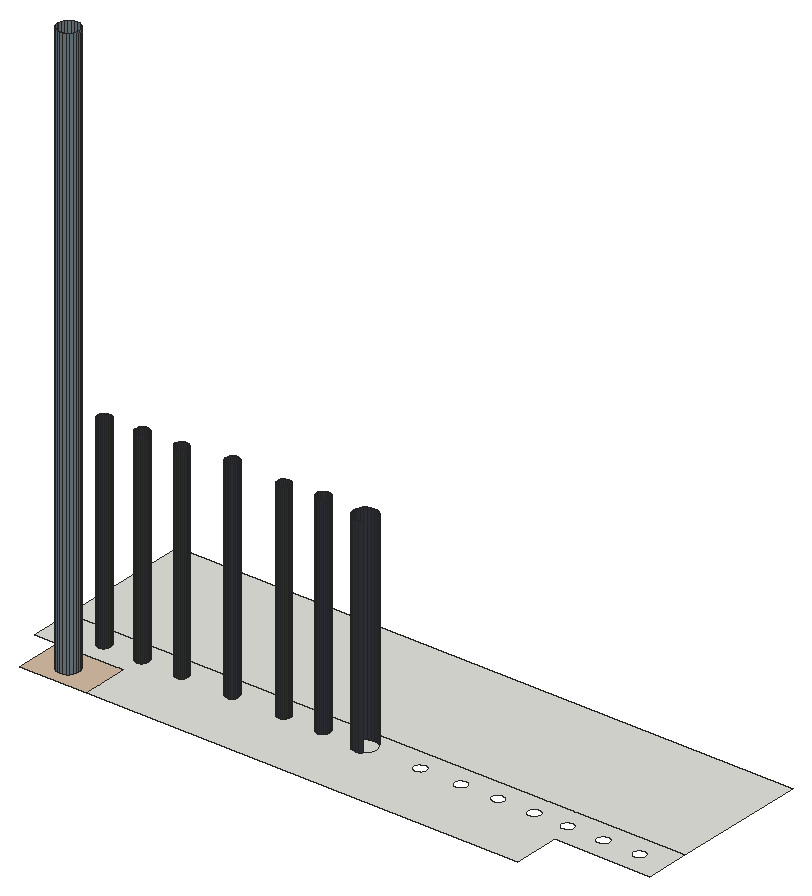
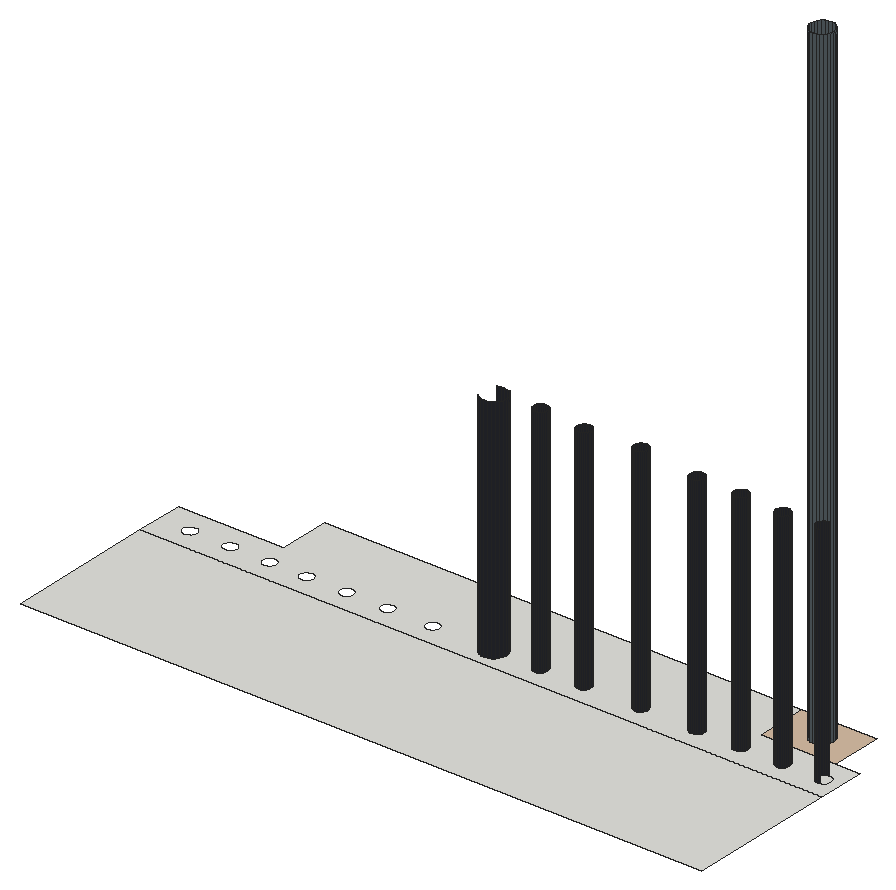
# SketchUp Ruby script. Lengths in inches.
U = 1.inch
M = Sketchup.active_model
def pt(a) = Geom::Point3d.new(a.map { |v| v * U })
def face(e, loops, mat)
  f = e.add_face(loops[0].map { |a| pt(a) })
  loops[1..].each { |l| e.add_face(l.map { |a| pt(a) }).erase! }
  f.material = f.back_material = mat if mat
  f
end
# faces: each face lists its corners as indices into pts; further lists are holes
def faces(e, pts, list, mat = nil) = list.each { |f| face(e, (f[0].is_a?(Array) ? f : [f]).map { |l| l.map { |i| pts[i] } }, mat) }
# xy, xz, yz: faces in a plane at the given z, y or x. An outline is a flat list of corners, or four numbers for a rectangle; further outlines are holes
def ring(l) = l.size == 4 ? [[l[0], l[1]], [l[2], l[1]], [l[2], l[3]], [l[0], l[3]]] : l.each_slice(2).to_a
def flat(e, list, mat, &to3) = list.each { |f| face(e, (f[0].is_a?(Array) ? f : [f]).map { |l| ring(l).map { |u, v| to3.(u, v) } }, mat) }
def xy(e, z, list, mat = nil) = flat(e, list, mat) { |x, y| [x, y, z] }
def xz(e, y, list, mat = nil) = flat(e, list, mat) { |x, z| [x, y, z] }
def yz(e, x, list, mat = nil) = flat(e, list, mat) { |y, z| [x, y, z] }
def lines(e, pts, list) = list.each { |a, b| e.add_line(pt(pts[a]), pt(pts[b])) }
# prism: a flat outline (further loops are holes) pulled along v
def prism(e, loops, v, mat = nil)
  f = face(e, loops, mat); d = Geom::Vector3d.new(v.map { |x| x * U })
  f.pushpull(f.normal.samedirection?(d) ? d.length : -d.length)
end
def box(e, o, s, mat = nil) = prism(e, [[o, [o[0] + s[0], o[1], o[2]], [o[0] + s[0], o[1] + s[1], o[2]], [o[0], o[1] + s[1], o[2]]]], [0, 0, s[2]], mat)
def at(x, y, z, deg = 0) = Geom::Transformation.translation(pt([x, y, z])) * Geom::Transformation.rotation(ORIGIN, Z_AXIS, deg.degrees)
def axes(o, x, y, z) = Geom::Transformation.new([*x, 0, *y, 0, *z, 0, *pt(o).to_a, 1])
def part(name) = M.definitions.add(name)
# library, detail: a bought-in or finely detailed component or shape, given as its bounding box
def library(name, o, s) = part(name).tap { |d| box(d.entities, o, s) }
def detail(e, o, s) = box(e.add_group.entities, o, s)
def put(e, d, t, mat = nil) = e.add_instance(d, t).tap { |i| i.material = mat if mat }
def group(e, t, mat = nil) = e.add_group.tap { |g| g.transformation = t; g.material = mat if mat }.entities
root = M.entities
M.materials.add("[Formica Laminate Dark]").color = [50, 53, 60]
M.materials.add("[Formica Laminate Light]").color = [213, 189, 164]
M.materials.add("[Formica Speckled Grey]").color = [112, 125, 132]
xy(root,479.47,[[[305.49,83.42,364.3,83.42,364.3,89.73,377.32,89.73,377.32,95.64,293.32,95.64,293.32,89.73,305.49,89.73],[335.9,91.32,335.49,91.37,335.11,91.53,334.79,91.78,334.54,92.1,334.39,92.48,334.33,92.88,334.39,93.28,334.54,93.66,334.79,93.99,335.11,94.23,335.49,94.39,335.9,94.44,336.3,94.39,336.68,94.23,337,93.99,337.25,93.66,337.41,93.28,337.46,92.88,337.41,92.48,337.25,92.1,337,91.78,336.68,91.53,336.3,91.37],[317.9,91.9,317.68,91.93,317.47,92.02,317.28,92.16,317.15,92.34,317.06,92.55,317.03,92.78,317.06,93.01,317.15,93.22,317.28,93.4,317.47,93.54,317.68,93.625,317.9,93.65,318.13,93.625,318.34,93.54,318.52,93.4,318.66,93.22,318.75,93.01,318.78,92.78,318.75,92.55,318.66,92.34,318.52,92.16,318.34,92.02,318.13,91.93],[343.53,91.9,343.3,91.93,343.09,92.02,342.91,92.16,342.77,92.34,342.68,92.55,342.65,92.78,342.68,93.01,342.77,93.22,342.91,93.4,343.09,93.54,343.3,93.625,343.53,93.65,343.75,93.625,343.97,93.54,344.15,93.4,344.29,93.22,344.375,93.01,344.4,92.78,344.375,92.55,344.29,92.34,344.15,92.16,343.97,92.02,343.75,91.93],[373.47,91.9,373.24,91.93,373.03,92.02,372.85,92.16,372.71,92.34,372.62,92.55,372.59,92.78,372.62,93.01,372.71,93.22,372.85,93.4,373.03,93.54,373.24,93.625,373.47,93.65,373.69,93.625,373.9,93.54,374.08,93.4,374.22,93.22,374.3125,93.01,374.34,92.78,374.3125,92.55,374.22,92.34,374.08,92.16,373.9,92.02,373.69,91.93],[349.09,91.9,348.86,91.93,348.65,92.02,348.47,92.16,348.33,92.34,348.25,92.55,348.22,92.78,348.25,93.01,348.33,93.22,348.47,93.4,348.65,93.54,348.86,93.625,349.09,93.65,349.32,93.625,349.53,93.54,349.71,93.4,349.85,93.22,349.9375,93.01,349.97,92.78,349.9375,92.55,349.85,92.34,349.71,92.16,349.53,92.02,349.32,91.93],[368.53,91.9,368.3,91.93,368.09,92.02,367.91,92.16,367.77,92.34,367.68,92.55,367.65,92.78,367.68,93.01,367.77,93.22,367.91,93.4,368.09,93.54,368.3,93.625,368.53,93.65,368.75,93.625,368.97,93.54,369.15,93.4,369.29,93.22,369.375,93.01,369.4,92.78,369.375,92.55,369.29,92.34,369.15,92.16,368.97,92.02,368.75,91.93],[354.15,91.9,353.93,91.93,353.72,92.02,353.53,92.16,353.4,92.34,353.31,92.55,353.28,92.78,353.31,93.01,353.4,93.22,353.53,93.4,353.72,93.54,353.93,93.625,354.15,93.65,354.38,93.625,354.59,93.54,354.77,93.4,354.91,93.22,355,93.01,355.03,92.78,355,92.55,354.91,92.34,354.77,92.16,354.59,92.02,354.38,91.93],[363.65,91.9,363.43,91.93,363.22,92.02,363.03,92.16,362.9,92.34,362.81,92.55,362.78,92.78,362.81,93.01,362.9,93.22,363.03,93.4,363.22,93.54,363.43,93.625,363.65,93.65,363.88,93.625,364.09,93.54,364.27,93.4,364.41,93.22,364.5,93.01,364.53,92.78,364.5,92.55,364.41,92.34,364.27,92.16,364.09,92.02,363.88,91.93],[359.09,91.9,358.86,91.93,358.65,92.02,358.47,92.16,358.33,92.34,358.25,92.55,358.22,92.78,358.25,93.01,358.33,93.22,358.47,93.4,358.65,93.54,358.86,93.625,359.09,93.65,359.32,93.625,359.53,93.54,359.71,93.4,359.85,93.22,359.9375,93.01,359.97,92.78,359.9375,92.55,359.85,92.34,359.71,92.16,359.53,92.02,359.32,91.93],[295.4,91.9,295.18,91.93,294.97,92.02,294.78,92.16,294.65,92.34,294.56,92.55,294.53,92.78,294.56,93.01,294.65,93.22,294.78,93.4,294.97,93.54,295.18,93.625,295.4,93.65,295.63,93.625,295.84,93.54,296.02,93.4,296.16,93.22,296.25,93.01,296.28,92.78,296.25,92.55,296.16,92.34,296.02,92.16,295.84,92.02,295.63,91.93],[330.28,91.9,330.05,91.93,329.84,92.02,329.66,92.16,329.52,92.34,329.43,92.55,329.4,92.78,329.43,93.01,329.52,93.22,329.66,93.4,329.84,93.54,330.05,93.625,330.28,93.65,330.5,93.625,330.72,93.54,330.9,93.4,331.04,93.22,331.125,93.01,331.15,92.78,331.125,92.55,331.04,92.34,330.9,92.16,330.72,92.02,330.5,91.93],[300.4,91.9,300.18,91.93,299.97,92.02,299.78,92.16,299.65,92.34,299.56,92.55,299.53,92.78,299.56,93.01,299.65,93.22,299.78,93.4,299.97,93.54,300.18,93.625,300.4,93.65,300.63,93.625,300.84,93.54,301.02,93.4,301.16,93.22,301.25,93.01,301.28,92.78,301.25,92.55,301.16,92.34,301.02,92.16,300.84,92.02,300.63,91.93],[324.9,91.9,324.68,91.93,324.47,92.02,324.28,92.16,324.15,92.34,324.06,92.55,324.03,92.78,324.06,93.01,324.15,93.22,324.28,93.4,324.47,93.54,324.68,93.625,324.9,93.65,325.13,93.625,325.34,93.54,325.52,93.4,325.66,93.22,325.75,93.01,325.78,92.78,325.75,92.55,325.66,92.34,325.52,92.16,325.34,92.02,325.13,91.93],[305.59,91.9,305.36,91.93,305.15,92.02,304.97,92.16,304.83,92.34,304.75,92.55,304.72,92.78,304.75,93.01,304.83,93.22,304.97,93.4,305.15,93.54,305.36,93.625,305.59,93.65,305.82,93.625,306.03,93.54,306.21,93.4,306.35,93.22,306.4375,93.01,306.47,92.78,306.4375,92.55,306.35,92.34,306.21,92.16,306.03,92.02,305.82,91.93],[310.97,91.9,310.74,91.93,310.53,92.02,310.35,92.16,310.21,92.34,310.12,92.55,310.09,92.78,310.12,93.01,310.21,93.22,310.35,93.4,310.53,93.54,310.74,93.625,310.97,93.65,311.19,93.625,311.4,93.54,311.58,93.4,311.72,93.22,311.8125,93.01,311.84,92.78,311.8125,92.55,311.72,92.34,311.58,92.16,311.4,92.02,311.19,91.93]],[300.64,84.97,300.26,85.02,299.92,85.17,299.62,85.4,299.39,85.69,299.25,86.04,299.2,86.41,299.25,86.78,299.39,87.13,299.62,87.43,299.92,87.66,300.26,87.8,300.64,87.85,301.01,87.8,301.36,87.66,301.65,87.43,301.88,87.13,302.03,86.78,302.07,86.41,302.03,86.04,301.88,85.69,301.65,85.4,301.36,85.17,301.01,85.02],[335.9,91.32,335.49,91.37,335.11,91.53,334.79,91.78,334.54,92.1,334.39,92.48,334.33,92.88,334.39,93.28,334.54,93.66,334.79,93.99,335.11,94.23,335.49,94.39,335.9,94.44,336.3,94.39,336.68,94.23,337,93.99,337.25,93.66,337.41,93.28,337.46,92.88,337.41,92.48,337.25,92.1,337,91.78,336.68,91.53,336.3,91.37],[295.4,91.9,295.18,91.93,294.97,92.02,294.78,92.16,294.65,92.34,294.56,92.55,294.53,92.78,294.56,93.01,294.65,93.22,294.78,93.4,294.97,93.54,295.18,93.625,295.4,93.65,295.63,93.625,295.84,93.54,296.02,93.4,296.16,93.22,296.25,93.01,296.28,92.78,296.25,92.55,296.16,92.34,296.02,92.16,295.84,92.02,295.63,91.93],[300.4,91.9,300.18,91.93,299.97,92.02,299.78,92.16,299.65,92.34,299.56,92.55,299.53,92.78,299.56,93.01,299.65,93.22,299.78,93.4,299.97,93.54,300.18,93.625,300.4,93.65,300.63,93.625,300.84,93.54,301.02,93.4,301.16,93.22,301.25,93.01,301.28,92.78,301.25,92.55,301.16,92.34,301.02,92.16,300.84,92.02,300.63,91.93],
  [305.59,91.9,305.36,91.93,305.15,92.02,304.97,92.16,304.83,92.34,304.75,92.55,304.72,92.78,304.75,93.01,304.83,93.22,304.97,93.4,305.15,93.54,305.36,93.625,305.59,93.65,305.82,93.625,306.03,93.54,306.21,93.4,306.35,93.22,306.4375,93.01,306.47,92.78,306.4375,92.55,306.35,92.34,306.21,92.16,306.03,92.02,305.82,91.93],[310.97,91.9,310.74,91.93,310.53,92.02,310.35,92.16,310.21,92.34,310.12,92.55,310.09,92.78,310.12,93.01,310.21,93.22,310.35,93.4,310.53,93.54,310.74,93.625,310.97,93.65,311.19,93.625,311.4,93.54,311.58,93.4,311.72,93.22,311.8125,93.01,311.84,92.78,311.8125,92.55,311.72,92.34,311.58,92.16,311.4,92.02,311.19,91.93],[317.9,91.9,317.68,91.93,317.47,92.02,317.28,92.16,317.15,92.34,317.06,92.55,317.03,92.78,317.06,93.01,317.15,93.22,317.28,93.4,317.47,93.54,317.68,93.625,317.9,93.65,318.13,93.625,318.34,93.54,318.52,93.4,318.66,93.22,318.75,93.01,318.78,92.78,318.75,92.55,318.66,92.34,318.52,92.16,318.34,92.02,318.13,91.93],[324.9,91.9,324.68,91.93,324.47,92.02,324.28,92.16,324.15,92.34,324.06,92.55,324.03,92.78,324.06,93.01,324.15,93.22,324.28,93.4,324.47,93.54,324.68,93.625,324.9,93.65,325.13,93.625,325.34,93.54,325.52,93.4,325.66,93.22,325.75,93.01,325.78,92.78,325.75,92.55,325.66,92.34,325.52,92.16,325.34,92.02,325.13,91.93],[330.28,91.9,330.05,91.93,329.84,92.02,329.66,92.16,329.52,92.34,329.43,92.55,329.4,92.78,329.43,93.01,329.52,93.22,329.66,93.4,329.84,93.54,330.05,93.625,330.28,93.65,330.5,93.625,330.72,93.54,330.9,93.4,331.04,93.22,331.125,93.01,331.15,92.78,331.125,92.55,331.04,92.34,330.9,92.16,330.72,92.02,330.5,91.93],
  [293.32,95.64,377.32,114.1]])
xy(root,479.47,[[[296.37,83.42,305.49,89.73],[300.64,84.97,300.26,85.02,299.92,85.17,299.62,85.4,299.39,85.69,299.25,86.04,299.2,86.41,299.25,86.78,299.39,87.13,299.62,87.43,299.92,87.66,300.26,87.8,300.64,87.85,301.01,87.8,301.36,87.66,301.65,87.43,301.88,87.13,302.03,86.78,302.07,86.41,302.03,86.04,301.88,85.69,301.65,85.4,301.36,85.17,301.01,85.02]]],"[Formica Laminate Light]")
p = [[299.92,85.17,479.47],[300.26,85.02,479.47],[300.26,85.02,557.86],[299.92,85.17,557.86],[300.64,84.97,479.47],[300.64,84.97,557.86],
  [301.01,85.02,479.47],[301.01,85.02,557.86],[301.36,85.17,479.47],[301.36,85.17,557.86],[299.62,85.4,479.47],[299.62,85.4,557.86],
  [301.65,85.4,479.47],[301.65,85.4,557.86],[299.39,85.69,479.47],[299.39,85.69,557.86],[301.88,85.69,479.47],[301.88,85.69,557.86],
  [299.25,86.04,479.47],[299.25,86.04,557.86],[302.03,86.04,479.47],[302.03,86.04,557.86],[299.2,86.41,479.47],[299.2,86.41,557.86],
  [302.07,86.41,479.47],[302.07,86.41,557.86],[299.25,86.78,479.47],[299.25,86.78,557.86],[302.03,86.78,479.47],[302.03,86.78,557.86],
  [299.39,87.13,479.47],[299.39,87.13,557.86],[301.88,87.13,479.47],[301.88,87.13,557.86],[299.62,87.43,479.47],[299.62,87.43,557.86],
  [301.65,87.43,479.47],[301.65,87.43,557.86],[299.92,87.66,479.47],[299.92,87.66,557.86],[301.36,87.66,479.47],[301.36,87.66,557.86],
  [300.26,87.8,479.47],[300.26,87.8,557.86],[301.01,87.8,479.47],[301.01,87.8,557.86],[300.64,87.85,479.47],[300.64,87.85,557.86],
  [335.49,91.37,479.47],[335.9,91.32,479.47],[335.9,91.32,507.81],[335.49,91.37,507.81],[336.3,91.37,479.47],[336.3,91.37,507.81],
  [335.11,91.53,479.47],[335.11,91.53,507.81],[336.68,91.53,479.47],[336.68,91.53,507.81],[334.79,91.78,479.47],[334.79,91.78,507.81],
  [334.54,92.1,479.47],[334.54,92.1,507.81],[295.4,91.9,479.47],[295.63,91.93,479.47],[295.63,91.93,507.47],[295.4,91.9,507.47],
  [295.84,92.02,479.47],[295.84,92.02,507.47],[299.97,92.02,479.47],[300.18,91.93,479.47],[300.18,91.93,507.22],[299.97,92.02,507.22],
  [300.4,91.9,479.47],[300.4,91.9,507.22],[300.63,91.93,479.47],[300.63,91.93,507.22],[300.84,92.02,479.47],[300.84,92.02,507.22],
  [305.15,92.02,479.47],[305.36,91.93,479.47],[305.36,91.93,507.41],[305.15,92.02,507.41],[305.59,91.9,479.47],[305.59,91.9,507.41],
  [305.82,91.93,479.47],[305.82,91.93,507.41],[306.03,92.02,479.47],[306.03,92.02,507.41],[310.53,92.02,479.47],[310.74,91.93,479.47],
  [310.74,91.93,507.47],[310.53,92.02,507.47],[310.97,91.9,479.47],[310.97,91.9,507.47],[311.19,91.93,479.47],[311.19,91.93,507.47],
  [311.4,92.02,479.47],[311.4,92.02,507.47],[317.47,92.02,479.47],[317.68,91.93,479.47],[317.68,91.93,508.19],[317.47,92.02,508.19],
  [317.9,91.9,479.47],[317.9,91.9,508.19],[318.13,91.93,479.47],[318.13,91.93,508.19],[318.34,92.02,479.47],[318.34,92.02,508.19],
  [324.47,92.02,479.47],[324.68,91.93,479.47],[324.68,91.93,507.81],[324.47,92.02,507.81],[324.9,91.9,479.47],[324.9,91.9,507.81],
  [325.13,91.93,479.47],[325.13,91.93,507.81],[325.34,92.02,479.47],[325.34,92.02,507.81],[329.84,92.02,479.47],[330.05,91.93,479.47],
  [330.05,91.93,508.19],[329.84,92.02,508.19],[330.28,91.9,479.47],[330.28,91.9,508.19],[330.5,91.93,479.47],[330.5,91.93,508.19],
  [330.72,92.02,479.47],[330.72,92.02,508.19],[296.02,92.16,479.47],[296.02,92.16,507.47],[299.78,92.16,479.47],[299.78,92.16,507.22],
  [301.02,92.16,479.47],[301.02,92.16,507.22],[304.97,92.16,479.47],[304.97,92.16,507.41],[306.21,92.16,479.47],[306.21,92.16,507.41],
  [310.35,92.16,479.47],[310.35,92.16,507.47],[311.58,92.16,479.47],[311.58,92.16,507.47],[317.28,92.16,479.47],[317.28,92.16,508.19],
  [318.52,92.16,479.47],[318.52,92.16,508.19],[324.28,92.16,479.47],[324.28,92.16,507.81],[325.52,92.16,479.47],[325.52,92.16,507.81],
  [329.66,92.16,479.47],[329.66,92.16,508.19],[330.9,92.16,479.47],[330.9,92.16,508.19],[334.39,92.48,479.47],[334.39,92.48,507.81],
  [296.16,92.34,479.47],[296.16,92.34,507.47],[299.65,92.34,479.47],[299.65,92.34,507.22],[301.16,92.34,479.47],[301.16,92.34,507.22],
  [304.83,92.34,479.47],[304.83,92.34,507.41],[306.35,92.34,479.47],[306.35,92.34,507.41],[310.21,92.34,479.47],[310.21,92.34,507.47],
  [311.72,92.34,479.47],[311.72,92.34,507.47],[317.15,92.34,479.47],[317.15,92.34,508.19],[318.66,92.34,479.47],[318.66,92.34,508.19],
  [324.15,92.34,479.47],[324.15,92.34,507.81],[325.66,92.34,479.47],[325.66,92.34,507.81],[329.52,92.34,479.47],[329.52,92.34,508.19],
  [331.04,92.34,479.47],[331.04,92.34,508.19],[296.25,92.55,479.47],[296.25,92.55,507.47],[299.56,92.55,479.47],[299.56,92.55,507.22],
  [301.25,92.55,479.47],[301.25,92.55,507.22],[304.75,92.55,479.47],[304.75,92.55,507.41],[306.4375,92.55,479.47],[306.4375,92.55,507.41],
  [310.12,92.55,479.47],[310.12,92.55,507.47],[311.8125,92.55,479.47],[311.8125,92.55,507.47],[317.06,92.55,479.47],[317.06,92.55,508.19],
  [318.75,92.55,479.47],[318.75,92.55,508.19],[324.06,92.55,479.47],[324.06,92.55,507.81],[325.75,92.55,479.47],[325.75,92.55,507.81],
  [329.43,92.55,479.47],[329.43,92.55,508.19],[331.125,92.55,479.47],[331.125,92.55,508.19],[334.33,92.88,479.47],[334.33,92.88,507.81],
  [296.28,92.78,479.47],[296.28,92.78,507.47],[299.53,92.78,479.47],[299.53,92.78,507.22],[301.28,92.78,479.47],[301.28,92.78,507.22],
  [304.72,92.78,479.47],[304.72,92.78,507.41],[306.47,92.78,479.47],[306.47,92.78,507.41],[310.09,92.78,479.47],[310.09,92.78,507.47],
  [311.84,92.78,479.47],[311.84,92.78,507.47],[317.03,92.78,479.47],[317.03,92.78,508.19],[318.78,92.78,479.47],[318.78,92.78,508.19],
  [324.03,92.78,479.47],[324.03,92.78,507.81],[325.78,92.78,479.47],[325.78,92.78,507.81],[329.4,92.78,479.47],[329.4,92.78,508.19],
  [331.15,92.78,479.47],[331.15,92.78,508.19],[296.25,93.01,479.47],[296.25,93.01,507.47],[299.56,93.01,479.47],[299.56,93.01,507.22],
  [301.25,93.01,479.47],[301.25,93.01,507.22],[304.75,93.01,479.47],[304.75,93.01,507.41],[306.4375,93.01,479.47],[306.4375,93.01,507.41],
  [310.12,93.01,479.47],[310.12,93.01,507.47],[311.8125,93.01,479.47],[311.8125,93.01,507.47],[317.06,93.01,479.47],[317.06,93.01,508.19],
  [318.75,93.01,479.47],[318.75,93.01,508.19],[324.06,93.01,479.47],[324.06,93.01,507.81],[325.75,93.01,479.47],[325.75,93.01,507.81],
  [329.43,93.01,479.47],[329.43,93.01,508.19],[331.125,93.01,479.47],[331.125,93.01,508.19],[334.39,93.28,479.47],[334.39,93.28,507.81],
  [296.16,93.22,479.47],[296.16,93.22,507.47],[299.65,93.22,479.47],[299.65,93.22,507.22],[301.16,93.22,479.47],[301.16,93.22,507.22],
  [304.83,93.22,479.47],[304.83,93.22,507.41],[306.35,93.22,479.47],[306.35,93.22,507.41],[310.21,93.22,479.47],[310.21,93.22,507.47],
  [311.72,93.22,479.47],[311.72,93.22,507.47],[317.15,93.22,479.47],[317.15,93.22,508.19],[318.66,93.22,479.47],[318.66,93.22,508.19],
  [324.15,93.22,479.47],[324.15,93.22,507.81],[325.66,93.22,479.47],[325.66,93.22,507.81],[329.52,93.22,479.47],[329.52,93.22,508.19],
  [331.04,93.22,479.47],[331.04,93.22,508.19],[296.02,93.4,479.47],[296.02,93.4,507.47],[299.78,93.4,479.47],[299.78,93.4,507.22],
  [301.02,93.4,479.47],[301.02,93.4,507.22],[304.97,93.4,479.47],[304.97,93.4,507.41],[306.21,93.4,479.47],[306.21,93.4,507.41],
  [310.35,93.4,479.47],[310.35,93.4,507.47],[311.58,93.4,479.47],[311.58,93.4,507.47],[317.28,93.4,479.47],[317.28,93.4,508.19],
  [318.52,93.4,479.47],[318.52,93.4,508.19],[324.28,93.4,479.47],[324.28,93.4,507.81],[325.52,93.4,479.47],[325.52,93.4,507.81],
  [329.66,93.4,479.47],[329.66,93.4,508.19],[330.9,93.4,479.47],[330.9,93.4,508.19],[334.54,93.66,479.47],[334.54,93.66,507.81],
  [295.84,93.54,479.47],[295.84,93.54,507.47],[299.97,93.54,479.47],[299.97,93.54,507.22],[300.84,93.54,479.47],[300.84,93.54,507.22],
  [305.15,93.54,479.47],[305.15,93.54,507.41],[306.03,93.54,479.47],[306.03,93.54,507.41],[310.53,93.54,479.47],[310.53,93.54,507.47],
  [311.4,93.54,479.47],[311.4,93.54,507.47],[317.47,93.54,479.47],[317.47,93.54,508.19],[318.34,93.54,479.47],[318.34,93.54,508.19],
  [324.47,93.54,479.47],[324.47,93.54,507.81],[325.34,93.54,479.47],[325.34,93.54,507.81],[329.84,93.54,479.47],[329.84,93.54,508.19],
  [330.72,93.54,479.47],[330.72,93.54,508.19],[295.63,93.625,479.47],[295.63,93.625,507.47],[300.18,93.625,479.47],[300.18,93.625,507.22],
  [300.63,93.625,479.47],[300.63,93.625,507.22],[305.36,93.625,479.47],[305.36,93.625,507.41],[305.82,93.625,479.47],[305.82,93.625,507.41],
  [310.74,93.625,479.47],[310.74,93.625,507.47],[311.19,93.625,479.47],[311.19,93.625,507.47],[317.68,93.625,479.47],[317.68,93.625,508.19],
  [318.13,93.625,479.47],[318.13,93.625,508.19],[324.68,93.625,479.47],[324.68,93.625,507.81],[325.13,93.625,479.47],[325.13,93.625,507.81],
  [330.05,93.625,479.47],[330.05,93.625,508.19],[330.5,93.625,479.47],[330.5,93.625,508.19],[295.4,93.65,479.47],[295.18,93.625,479.47],
  [295.18,93.625,507.47],[295.4,93.65,507.47],[300.4,93.65,479.47],[300.4,93.65,507.22],[305.59,93.65,479.47],[305.59,93.65,507.41],
  [310.97,93.65,479.47],[310.97,93.65,507.47],[317.9,93.65,479.47],[317.9,93.65,508.19],[324.9,93.65,479.47],[324.9,93.65,507.81],
  [330.28,93.65,479.47],[330.28,93.65,508.19],[334.79,93.99,479.47],[334.79,93.99,507.81],[335.11,94.23,479.47],[335.08,94.21,507.81],
  [335.11,94.23,507.81],[337,93.99,479.47],[336.68,94.23,479.47],[336.68,94.23,507.81],[336.71,94.21,507.81],[337,93.99,507.81],
  [335.49,94.39,479.47],[335.49,94.39,507.81],[336.3,94.39,479.47],[336.3,94.39,507.81],[335.9,94.44,479.47],[335.9,94.44,507.81]]
faces(root,p,[[0,1,2,3],[1,4,5,2],[4,6,7,5],[6,8,9,7],[10,0,3,11],[8,12,13,9],[14,10,11,15],[12,16,17,13],
  [18,14,15,19],[16,20,21,17],[22,18,19,23],[20,24,25,21],[26,22,23,27],[24,28,29,25],[30,26,27,31],[28,32,33,29],
  [34,30,31,35],[32,36,37,33],[38,34,35,39],[36,40,41,37],[42,38,39,43],[40,44,45,41],[46,42,43,47],[44,46,47,45]],"[Formica Speckled Grey]")
faces(root,p,[[48,49,50,51],[49,52,53,50],[54,48,51,55],[52,56,57,53],[58,54,55,59],[60,58,59,61],[62,63,64,65],[63,66,67,64],
  [68,69,70,71],[69,72,73,70],[72,74,75,73],[74,76,77,75],[78,79,80,81],[79,82,83,80],[82,84,85,83],[84,86,87,85],
  [88,89,90,91],[89,92,93,90],[92,94,95,93],[94,96,97,95],[98,99,100,101],[99,102,103,100],[102,104,105,103],[104,106,107,105],
  [108,109,110,111],[109,112,113,110],[112,114,115,113],[114,116,117,115],[118,119,120,121],[119,122,123,120],[122,124,125,123],[124,126,127,125],
  [66,128,129,67],[130,68,71,131],[76,132,133,77],[134,78,81,135],[86,136,137,87],[138,88,91,139],[96,140,141,97],[142,98,101,143],
  [106,144,145,107],[146,108,111,147],[116,148,149,117],[150,118,121,151],[126,152,153,127],[154,60,61,155],[128,156,157,129],[158,130,131,159],
  [132,160,161,133],[162,134,135,163],[136,164,165,137],[166,138,139,167],[140,168,169,141],[170,142,143,171],[144,172,173,145],[174,146,147,175],
  [148,176,177,149],[178,150,151,179],[152,180,181,153],[156,182,183,157],[184,158,159,185],[160,186,187,161],[188,162,163,189],[164,190,191,165],
  [192,166,167,193],[168,194,195,169],[196,170,171,197],[172,198,199,173],[200,174,175,201],[176,202,203,177],[204,178,179,205],[180,206,207,181],
  [208,154,155,209],[182,210,211,183],[212,184,185,213],[186,214,215,187],[216,188,189,217],[190,218,219,191],[220,192,193,221],[194,222,223,195],
  [224,196,197,225],[198,226,227,199],[228,200,201,229],[202,230,231,203],[232,204,205,233],[206,234,235,207],[210,236,237,211],[238,212,213,239],
  [214,240,241,215],[242,216,217,243],[218,244,245,219],[246,220,221,247],[222,248,249,223],[250,224,225,251],[226,252,253,227],[254,228,229,255],
  [230,256,257,231],[258,232,233,259],[234,260,261,235],[262,208,209,263],[236,264,265,237],[266,238,239,267],[240,268,269,241],[270,242,243,271],
  [244,272,273,245],[274,246,247,275],[248,276,277,249],[278,250,251,279],[252,280,281,253],[282,254,255,283],[256,284,285,257],[286,258,259,287],
  [260,288,289,261],[264,290,291,265],[292,266,267,293],[268,294,295,269],[296,270,271,297],[272,298,299,273],[300,274,275,301],[276,302,303,277],
  [304,278,279,305],[280,306,307,281],[308,282,283,309],[284,310,311,285],[312,286,287,313],[288,314,315,289],[316,262,263,317],[290,318,319,291],
  [320,292,293,321],[294,322,323,295],[324,296,297,325],[298,326,327,299],[328,300,301,329],[302,330,331,303],[332,304,305,333],[306,334,335,307],
  [336,308,309,337],[310,338,339,311],[340,312,313,341],[314,342,343,315],[318,344,345,319],[346,320,321,347],[322,348,349,323],[350,324,325,351],
  [326,352,353,327],[354,328,329,355],[330,356,357,331],[358,332,333,359],[334,360,361,335],[362,336,337,363],[338,364,365,339],[366,340,341,367],
  [342,368,369,343],[370,371,372,373],[344,370,373,345],[374,346,347,375],[348,374,375,349],[376,350,351,377],[352,376,377,353],[378,354,355,379],
  [356,378,379,357],[380,358,359,381],[360,380,381,361],[382,362,363,383],[364,382,383,365],[384,366,367,385],[368,384,385,369],[386,316,317,387],
  [388,386,387,389,390],[391,392,393,394,395],[396,388,390,397],[392,398,399,393],[400,396,397,401],[398,400,401,399]],"[Formica Laminate Dark]")
